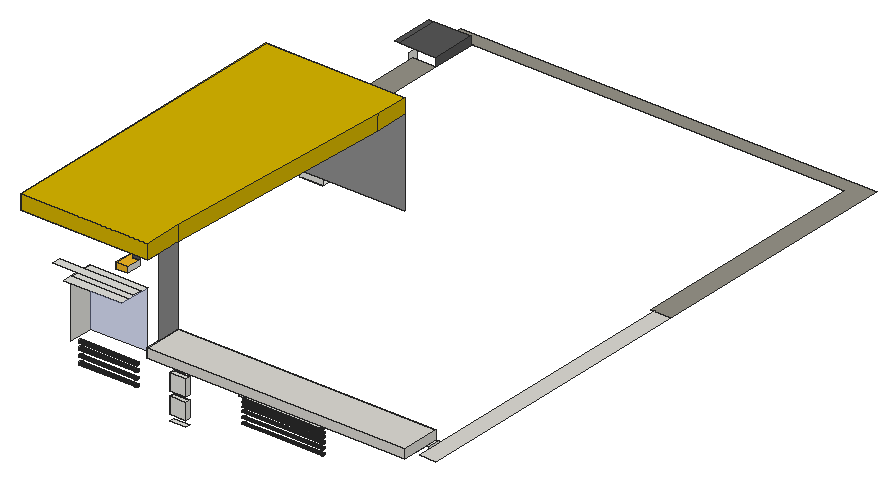
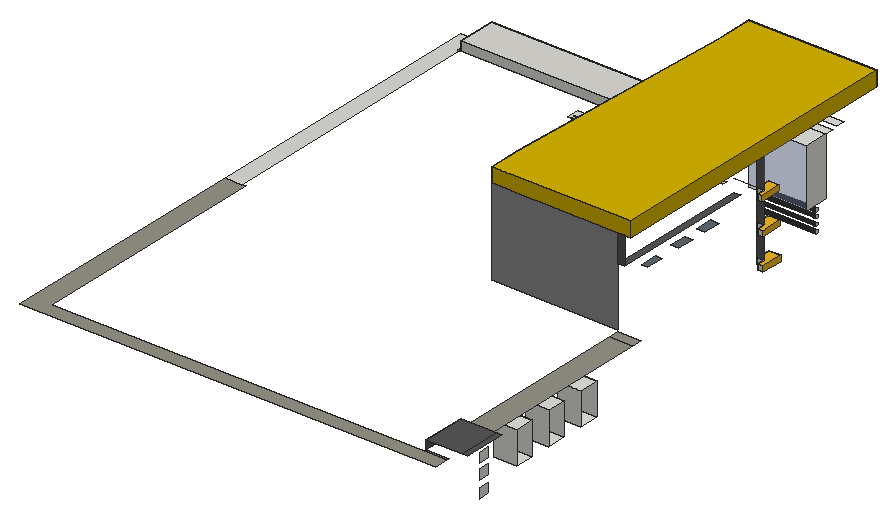
# SketchUp Ruby script. Lengths in inches.
U = 1.inch
M = Sketchup.active_model
def pt(a) = Geom::Point3d.new(a.map { |v| v * U })
def face(e, loops, mat)
  f = e.add_face(loops[0].map { |a| pt(a) })
  loops[1..].each { |l| e.add_face(l.map { |a| pt(a) }).erase! }
  f.material = f.back_material = mat if mat
  f
end
# faces: each face lists its corners as indices into pts; further lists are holes
def faces(e, pts, list, mat = nil) = list.each { |f| face(e, (f[0].is_a?(Array) ? f : [f]).map { |l| l.map { |i| pts[i] } }, mat) }
# xy, xz, yz: faces in a plane at the given z, y or x. An outline is a flat list of corners, or four numbers for a rectangle; further outlines are holes
def ring(l) = l.size == 4 ? [[l[0], l[1]], [l[2], l[1]], [l[2], l[3]], [l[0], l[3]]] : l.each_slice(2).to_a
def flat(e, list, mat, &to3) = list.each { |f| face(e, (f[0].is_a?(Array) ? f : [f]).map { |l| ring(l).map { |u, v| to3.(u, v) } }, mat) }
def xy(e, z, list, mat = nil) = flat(e, list, mat) { |x, y| [x, y, z] }
def xz(e, y, list, mat = nil) = flat(e, list, mat) { |x, z| [x, y, z] }
def yz(e, x, list, mat = nil) = flat(e, list, mat) { |y, z| [x, y, z] }
def lines(e, pts, list) = list.each { |a, b| e.add_line(pt(pts[a]), pt(pts[b])) }
# prism: a flat outline (further loops are holes) pulled along v
def prism(e, loops, v, mat = nil)
  f = face(e, loops, mat); d = Geom::Vector3d.new(v.map { |x| x * U })
  f.pushpull(f.normal.samedirection?(d) ? d.length : -d.length)
end
def box(e, o, s, mat = nil) = prism(e, [[o, [o[0] + s[0], o[1], o[2]], [o[0] + s[0], o[1] + s[1], o[2]], [o[0], o[1] + s[1], o[2]]]], [0, 0, s[2]], mat)
def at(x, y, z, deg = 0) = Geom::Transformation.translation(pt([x, y, z])) * Geom::Transformation.rotation(ORIGIN, Z_AXIS, deg.degrees)
def axes(o, x, y, z) = Geom::Transformation.new([*x, 0, *y, 0, *z, 0, *pt(o).to_a, 1])
def part(name) = M.definitions.add(name)
# library, detail: a bought-in or finely detailed component or shape, given as its bounding box
def library(name, o, s) = part(name).tap { |d| box(d.entities, o, s) }
def detail(e, o, s) = box(e.add_group.entities, o, s)
def put(e, d, t, mat = nil) = e.add_instance(d, t).tap { |i| i.material = mat if mat }
def group(e, t, mat = nil) = e.add_group.tap { |g| g.transformation = t; g.material = mat if mat }.entities
root = M.entities
M.materials.add("[0045_Goldenrod]").color = [239, 181, 35]
M.materials.add("[0046_Gold]1").color = [214, 180, 0]
M.materials.add("[Color M04]").color = [142, 142, 142]
M.materials.add("[Color M06]").color = [86, 86, 86]
M.materials.add("[Color M07]").color = [58, 58, 58]
M.materials.add("[Formica Graystone]").color = [149, 146, 135]
M.materials.add("[Formica Speckled Grey]").color = [94, 105, 111]
M.materials.add("[Terrazzo Tile Light]").color = [219, 217, 210]
M.materials.add("[Translucent Glass Sky Reflection]").color = [126, 138, 183]
M.materials["[Translucent Glass Sky Reflection]"].alpha = 0.52
box(root,[220.22,108.25,417.34],[19.63,5.9375,19.63])
box(root,[220.22,108.25,443.22],[19.63,5.9375,19.62])
xy(root,409.78,[[220.22,108.25,239.85,114.1875]])
xy(root,414.79,[[25.28,551.74,53.375,575.93],[25.28,600.93,53.375,625.12],[25.28,649.81,53.375,673.99]])
xy(root,445.19,[[[280.22,138.52,379.09,153.42],[329.08,144.78,329.38,144.82,329.67,144.9375,329.91,145.125,330.1,145.37,330.22,145.66,330.26,145.96,330.22,146.27,330.1,146.56,329.91,146.8,329.67,146.99,329.38,147.11,329.08,147.15,328.77,147.11,328.48,146.99,328.24,146.8,328.05,146.56,327.93,146.27,327.89,145.96,327.93,145.66,328.05,145.37,328.24,145.125,328.48,144.9375,328.77,144.82]]])
xy(root,449.66,[[38.625,253.03,38.625,280.03,45.3125,280.03,45.3125,270.46,53.375,270.46,53.375,253.03]],"[0045_Goldenrod]")
xy(root,454.59,[[25.28,551.74,53.375,575.93],[25.28,600.93,53.375,625.12],[25.28,649.81,53.375,673.99]])
xy(root,456.47,[[38.625,253.03,53.375,253.03,53.375,270.46,45.3125,270.46,45.3125,280.03,38.625,280.03]],"[0045_Goldenrod]")
xy(root,468.5,[[25.28,483.625,53.375,495.58],[509.21,483.625,533.375,483.625,533.375,797.6875,25.28,797.6875,25.28,779.875,509.21,779.875],[25.28,495.58,53.375,724.47],[25.28,777.2,53.375,779.875]],"[Formica Graystone]")
xy(root,468.5,[[513.45,123.625,533.375,483.625]],"[Terrazzo Tile Light]")
xy(root,471,[[194.63,105.9375,276.16,114.1875],[276.16,105.9375,276.16,138.52,385.17,138.52,385.17,125.375,418.48,125.375,418.48,138.52,435.42,138.52,435.42,125.375,467.86,125.375,467.86,138.52,510.34,138.52,510.34,105.9375],[194.63,114.1875,276.16,123.625],[194.63,123.625,276.16,153.42],[385.17,125.375,418.48,138.52],
  [435.42,125.375,467.86,138.52],[276.16,138.52,510.34,153.42],[510.34,138.52,513.45,153.42]])
xy(root,479.1875,[[2.5625,724.47,8.375,777.2],[8.375,724.47,53.375,777.2]],"[Color M06]")
xy(root,481.9375,[[194.63,105.9375,510.34,153.42]],"[Terrazzo Tile Light]")
xy(root,488.34,[[39.4375,253.03,39.4375,280.03,45.3125,280.03,45.3125,270.46,53.375,270.46,53.375,253.03]],"[0045_Goldenrod]")
xy(root,495.16,[[39.4375,253.03,53.375,253.03,53.375,270.46,45.3125,270.46,45.3125,280.03,39.4375,280.03]],"[0045_Goldenrod]")
xy(root,515.31,[[87.31,112.625,158.23,123.625],[87.31,123.625,158.23,152]])
xy(root,519.67,[[53.375,329.18,63.8125,350.43],[53.375,369.37,62.6875,390.62],[53.375,417,60.4375,438.25]],"[Formica Speckled Grey]")
xy(root,526.41,[[40.5,253.03,40.5,280.03,45.3125,280.03,45.3125,270.46,53.375,270.46,53.375,253.03]],"[0045_Goldenrod]")
xy(root,529.3125,[[73.3,112.625,172.24,123.625]])
xy(root,533.22,[[40.5,253.03,53.375,253.03,53.375,270.46,45.3125,270.46,45.3125,280.03,40.5,280.03]],"[0045_Goldenrod]")
xy(root,543.2,[[45.3125,306.125,53.375,483.625]],"[Color M06]")
xy(root,577.3125,[[38.125,107.4375,53.375,136.75],[53.375,107.4375,194.63,123.625],[53.375,123.625,53.375,483.625,73.3,483.625,73.3,463.7,208.03,463.7,208.03,442.17,194.63,153.42,194.63,123.625],[38.125,136.75,45.75,151.32],[45.75,136.75,53.375,151.32],
  [38.125,151.32,53.375,169.81],[38.125,169.81,45.75,184.38],[45.75,169.81,53.375,184.38],[38.125,184.38,53.375,206.12],[38.125,206.12,45.75,220.7],
  [45.75,206.12,53.375,220.7],[38.125,220.7,53.375,270.46],[38.125,270.46,45.3125,483.625],[45.3125,270.46,53.375,483.625],[73.3,463.7,208.03,483.625]])
xy(root,595.5,[[38.125,107.4375,194.63,107.4375,194.63,153.42,208.03,442.17,208.03,483.625,38.125,483.625]],"[0046_Gold]1")
xz(root,105.9375,[[194.63,471,510.34,481.9375]],"[Terrazzo Tile Light]")
xz(root,107.4375,[[38.125,577.3125,194.63,595.5]],"[0046_Gold]1")
xz(root,152,[[87.31,444.16,158.23,515.31]],"[Translucent Glass Sky Reflection]")
xz(root,153.42,[[194.63,471,510.34,481.9375]])
xz(root,253.03,[[38.625,449.66,53.375,456.47],[39.4375,488.34,53.375,495.16],[40.5,526.41,53.375,533.22]],"[0045_Goldenrod]")
xz(root,270.46,[[45.3125,449.66,53.375,456.47],[45.3125,488.34,53.375,495.16],[45.3125,526.41,53.375,533.22]])
xz(root,270.46,[[45.3125,456.47,53.375,488.34],[45.3125,495.16,53.375,526.41],[45.3125,533.22,53.375,577.3125]],"[Color M06]")
xz(root,280.03,[[38.625,449.66,45.3125,456.47],[39.4375,488.34,45.3125,495.16],[40.5,526.41,45.3125,533.22]])
xz(root,483.625,[[38.125,577.3125,208.03,595.5]],"[0046_Gold]1")
xz(root,483.625,[[53.375,471,208.03,577.3125]],"[Color M04]")
xz(root,483.625,[[45.3125,543.2,53.375,577.3125]],"[Color M06]")
xz(root,551.74,[[25.28,414.79,53.375,454.59]])
xz(root,575.93,[[25.28,414.79,53.375,454.59]])
xz(root,600.93,[[25.28,414.79,53.375,454.59]])
xz(root,625.12,[[25.28,414.79,53.375,454.59]])
xz(root,649.81,[[25.28,414.79,53.375,454.59]])
xz(root,673.99,[[25.28,414.79,53.375,454.59]])
yz(root,2.5625,[[745.75,424.57,759.0625,436.32],[745.75,444.94,759.0625,456.69],[745.75,463.32,759.0625,475.07]])
yz(root,38.125,[[107.4375,577.3125,483.625,595.5]],"[0046_Gold]1")
yz(root,38.625,[[253.03,449.66,280.03,456.47]],"[0045_Goldenrod]")
yz(root,39.4375,[[253.03,488.34,280.03,495.16]],"[0045_Goldenrod]")
yz(root,40.5,[[253.03,526.41,280.03,533.22]],"[0045_Goldenrod]")
yz(root,45.3125,[[270.46,449.66,280.03,456.47],[270.46,488.34,280.03,495.16],[270.46,526.41,280.03,533.22]])
yz(root,53.375,[[253.03,449.66,270.46,456.47],[253.03,488.34,270.46,495.16],[253.03,526.41,270.46,533.22]])
yz(root,53.375,[[724.47,468.5,777.2,479.1875]],"[Color M06]")
yz(root,87.31,[[136.99,412.55,136.55,412.61,136.14,412.78,135.79,413.05,135.52,413.4,135.36,413.81,135.3,414.24,135.36,414.68,135.52,415.09,135.79,415.44,136.14,415.7,136.55,415.87,136.99,415.93,137.42,415.87,137.83,415.7,138.18,415.44,138.45,415.09,138.62,414.68,138.67,414.24,138.62,413.81,138.45,413.4,138.18,413.05,137.83,412.78,137.42,412.61],[136.99,420.74,136.55,420.8,136.14,420.97,135.79,421.24,135.52,421.59,135.36,421.99,135.3,422.43,135.36,422.87,135.52,423.27,135.79,423.62,136.14,423.89,136.55,424.06,136.99,424.12,137.42,424.06,137.83,423.89,138.18,423.62,138.45,423.27,138.62,422.87,138.67,422.43,138.62,421.99,138.45,421.59,138.18,421.24,137.83,420.97,137.42,420.8],[136.99,429.05,136.55,429.11,136.14,429.28,135.79,429.55,135.52,429.9,135.36,430.31,135.3,430.74,135.36,431.18,135.52,431.59,135.79,431.94,136.14,432.2,136.55,432.37,136.99,432.43,137.42,432.37,137.83,432.2,138.18,431.94,138.45,431.59,138.62,431.18,138.67,430.74,138.62,430.31,138.45,429.9,138.18,429.55,137.83,429.28,137.42,429.11],[136.99,436.55,136.55,436.61,136.14,436.78,135.79,437.05,135.52,437.4,135.36,437.81,135.3,438.24,135.36,438.68,135.52,439.09,135.79,439.44,136.14,439.7,136.55,439.87,136.99,439.93,137.42,439.87,137.83,439.7,138.18,439.44,138.45,439.09,138.62,438.68,138.67,438.24,138.62,437.81,138.45,437.4,138.18,437.05,137.83,436.78,137.42,436.61],[123.625,444.16,152,515.31]])
yz(root,194.63,[[123.625,471,153.42,481.9375]])
yz(root,194.63,[[107.4375,577.3125,153.42,595.5]],"[0046_Gold]1")
yz(root,194.63,[[123.625,481.9375,153.42,577.3125]],"[Color M04]")
yz(root,194.63,[[105.9375,471,123.625,481.9375]],"[Terrazzo Tile Light]")
yz(root,208.03,[[442.17,577.3125,483.625,595.5]],"[0046_Gold]1")
yz(root,280.22,[[145.61,411.18,145.26,411.23,144.93,411.37,144.64,411.59,144.42,411.87,144.29,412.2,144.24,412.56,144.29,412.92,144.42,413.25,144.64,413.53,144.93,413.75,145.26,413.89,145.61,413.93,145.97,413.89,146.3,413.75,146.59,413.53,146.81,413.25,146.94,412.92,146.99,412.56,146.94,412.2,146.81,411.87,146.59,411.59,146.3,411.37,145.97,411.23],[145.61,417.75,145.26,417.79,144.93,417.93,144.64,418.15,144.42,418.43,144.29,418.77,144.24,419.12,144.29,419.48,144.42,419.81,144.64,420.09,144.93,420.3125,145.26,420.45,145.61,420.5,145.97,420.45,146.3,420.3125,146.59,420.09,146.81,419.81,146.94,419.48,146.99,419.12,146.94,418.77,146.81,418.43,146.59,418.15,146.3,417.93,145.97,417.79],[145.61,424.12,145.26,424.17,144.93,424.31,144.64,424.52,144.42,424.81,144.29,425.14,144.24,425.5,144.29,425.85,144.42,426.18,144.64,426.47,144.93,426.6875,145.26,426.83,145.61,426.87,145.97,426.83,146.3,426.6875,146.59,426.47,146.81,426.18,146.94,425.85,146.99,425.5,146.94,425.14,146.81,424.81,146.59,424.52,146.3,424.31,145.97,424.17],[145.73,429.69,145.38,429.74,145.05,429.875,144.76,430.09,144.54,430.38,144.41,430.71,144.36,431.07,144.41,431.42,144.54,431.75,144.76,432.04,145.05,432.26,145.38,432.39,145.73,432.44,146.09,432.39,146.42,432.26,146.71,432.04,146.92,431.75,147.0625,431.42,147.11,431.07,147.0625,430.71,146.92,430.38,146.71,430.09,146.42,429.875,146.09,429.74],[145.73,434.63,145.38,434.67,145.05,434.8125,144.76,435.03,144.54,435.32,144.41,435.65,144.36,436,144.41,436.36,144.54,436.69,144.76,436.97,145.05,437.19,145.38,437.33,145.73,437.38,146.09,437.33,146.42,437.19,146.71,436.97,146.92,436.69,147.0625,436.36,147.11,436,147.0625,435.65,146.92,435.32,146.71,435.03,146.42,434.8125,146.09,434.67],
  [145.73,439.94,145.38,439.99,145.05,440.125,144.76,440.34,144.54,440.63,144.41,440.96,144.36,441.32,144.41,441.67,144.54,442,144.76,442.29,145.05,442.51,145.38,442.64,145.73,442.69,146.09,442.64,146.42,442.51,146.71,442.29,146.92,442,147.0625,441.67,147.11,441.32,147.0625,440.96,146.92,440.63,146.71,440.34,146.42,440.125,146.09,439.99]])
yz(root,510.34,[[105.9375,471,153.42,481.9375]],"[Terrazzo Tile Light]")
yz(root,513.45,[[138.52,468.5,153.42,471]])
p = [[280.22,144.93,411.37],[280.22,145.26,411.23],[379.09,145.26,411.23],[379.09,144.93,411.37],[280.22,145.61,411.18],[379.09,145.61,411.18],
  [280.22,145.97,411.23],[379.09,145.97,411.23],[280.22,146.3,411.37],[379.09,146.3,411.37],[280.22,144.64,411.59],[379.09,144.64,411.59],
  [280.22,146.59,411.59],[379.09,146.59,411.59],[280.22,144.42,411.87],[379.09,144.42,411.87],[280.22,146.81,411.87],[379.09,146.81,411.87],
  [280.22,144.29,412.2],[379.09,144.29,412.2],[280.22,146.94,412.2],[379.09,146.94,412.2],[280.22,144.24,412.56],[379.09,144.24,412.56],
  [280.22,146.99,412.56],[379.09,146.99,412.56],[87.31,136.14,412.78],[87.31,136.55,412.61],[158.23,136.55,412.61],[158.23,136.14,412.78],
  [87.31,136.99,412.55],[158.23,136.99,412.55],[87.31,137.42,412.61],[158.23,137.42,412.61],[87.31,137.83,412.78],[158.23,137.83,412.78],
  [280.22,144.29,412.92],[379.09,144.29,412.92],[280.22,146.94,412.92],[379.09,146.94,412.92],[87.31,135.79,413.05],[158.23,135.79,413.05],
  [87.31,138.18,413.05],[158.23,138.18,413.05],[280.22,144.42,413.25],[379.09,144.42,413.25],[280.22,146.81,413.25],[379.09,146.81,413.25],
  [87.31,135.52,413.4],[158.23,135.52,413.4],[87.31,138.45,413.4],[158.23,138.45,413.4],[280.22,144.64,413.53],[379.09,144.64,413.53],
  [280.22,146.59,413.53],[379.09,146.59,413.53],[87.31,135.36,413.81],[158.23,135.36,413.81],[87.31,138.62,413.81],[158.23,138.62,413.81],
  [280.22,144.93,413.75],[379.09,144.93,413.75],[280.22,146.3,413.75],[379.09,146.3,413.75],[87.31,135.3,414.24],[158.23,135.3,414.24],
  [87.31,138.67,414.24],[158.23,138.67,414.24],[280.22,145.26,413.89],[379.09,145.26,413.89],[280.22,145.97,413.89],[379.09,145.97,413.89],
  [280.22,145.61,413.93],[379.09,145.61,413.93],[87.31,135.36,414.68],[158.23,135.36,414.68],[87.31,138.62,414.68],[158.23,138.62,414.68],
  [87.31,135.52,415.09],[158.23,135.52,415.09],[87.31,138.45,415.09],[158.23,138.45,415.09],[87.31,135.79,415.44],[158.23,135.79,415.44],
  [87.31,138.18,415.44],[158.23,138.18,415.44],[87.31,136.14,415.7],[158.23,136.14,415.7],[87.31,137.83,415.7],[158.23,137.83,415.7],
  [87.31,136.55,415.87],[158.23,136.55,415.87],[87.31,137.42,415.87],[158.23,137.42,415.87],[87.31,136.99,415.93],[158.23,136.99,415.93],
  [280.22,145.26,417.79],[280.22,145.61,417.75],[379.09,145.61,417.75],[379.09,145.26,417.79],[280.22,145.97,417.79],[379.09,145.97,417.79],
  [280.22,144.93,417.93],[379.09,144.93,417.93],[280.22,146.3,417.93],[379.09,146.3,417.93],[280.22,144.64,418.15],[379.09,144.64,418.15],
  [280.22,146.59,418.15],[379.09,146.59,418.15],[280.22,144.42,418.43],[379.09,144.42,418.43],[280.22,146.81,418.43],[379.09,146.81,418.43],
  [280.22,144.29,418.77],[379.09,144.29,418.77],[280.22,146.94,418.77],[379.09,146.94,418.77],[280.22,144.24,419.12],[379.09,144.24,419.12],
  [280.22,146.99,419.12],[379.09,146.99,419.12],[280.22,144.29,419.48],[379.09,144.29,419.48],[280.22,146.94,419.48],[379.09,146.94,419.48],
  [280.22,144.42,419.81],[379.09,144.42,419.81],[280.22,146.81,419.81],[379.09,146.81,419.81],[280.22,144.64,420.09],[379.09,144.64,420.09],
  [280.22,146.59,420.09],[379.09,146.59,420.09],[280.22,144.93,420.3125],[379.09,144.93,420.3125],[280.22,146.3,420.3125],[379.09,146.3,420.3125],
  [280.22,145.26,420.45],[379.09,145.26,420.45],[280.22,145.97,420.45],[379.09,145.97,420.45],[280.22,145.61,420.5],[379.09,145.61,420.5],
  [87.31,136.55,420.8],[87.31,136.99,420.74],[158.23,136.99,420.74],[158.23,136.55,420.8],[87.31,137.42,420.8],[158.23,137.42,420.8],
  [87.31,136.14,420.97],[158.23,136.14,420.97],[87.31,137.83,420.97],[158.23,137.83,420.97],[87.31,135.79,421.24],[158.23,135.79,421.24],
  [87.31,138.18,421.24],[158.23,138.18,421.24],[87.31,135.52,421.59],[158.23,135.52,421.59],[87.31,138.45,421.59],[158.23,138.45,421.59],
  [87.31,135.36,421.99],[158.23,135.36,421.99],[87.31,138.62,421.99],[158.23,138.62,421.99],[87.31,135.3,422.43],[158.23,135.3,422.43],
  [87.31,138.67,422.43],[158.23,138.67,422.43],[87.31,135.36,422.87],[158.23,135.36,422.87],[87.31,138.62,422.87],[158.23,138.62,422.87],
  [87.31,135.52,423.27],[158.23,135.52,423.27],[87.31,138.45,423.27],[158.23,138.45,423.27],[87.31,135.79,423.62],[158.23,135.79,423.62],
  [87.31,138.18,423.62],[158.23,138.18,423.62],[87.31,136.14,423.89],[158.23,136.14,423.89],[87.31,137.83,423.89],[158.23,137.83,423.89],
  [87.31,136.55,424.06],[158.23,136.55,424.06],[87.31,137.42,424.06],[158.23,137.42,424.06],[87.31,136.99,424.12],[158.23,136.99,424.12],
  [280.22,145.26,424.17],[280.22,145.61,424.12],[379.09,145.61,424.12],[379.09,145.26,424.17],[280.22,145.97,424.17],[379.09,145.97,424.17],
  [280.22,144.93,424.31],[379.09,144.93,424.31],[280.22,146.3,424.31],[379.09,146.3,424.31],[280.22,144.64,424.52],[379.09,144.64,424.52],
  [280.22,146.59,424.52],[379.09,146.59,424.52],[280.22,144.42,424.81],[379.09,144.42,424.81],[280.22,146.81,424.81],[379.09,146.81,424.81],
  [280.22,144.29,425.14],[379.09,144.29,425.14],[280.22,146.94,425.14],[379.09,146.94,425.14],[280.22,144.24,425.5],[379.09,144.24,425.5],
  [280.22,146.99,425.5],[379.09,146.99,425.5],[280.22,144.29,425.85],[379.09,144.29,425.85],[280.22,146.94,425.85],[379.09,146.94,425.85],
  [280.22,144.42,426.18],[379.09,144.42,426.18],[280.22,146.81,426.18],[379.09,146.81,426.18],[280.22,144.64,426.47],[379.09,144.64,426.47],
  [280.22,146.59,426.47],[379.09,146.59,426.47],[280.22,144.93,426.6875],[379.09,144.93,426.6875],[280.22,146.3,426.6875],[379.09,146.3,426.6875],
  [280.22,145.26,426.83],[379.09,145.26,426.83],[280.22,145.97,426.83],[379.09,145.97,426.83],[280.22,145.61,426.87],[379.09,145.61,426.87],
  [87.31,136.14,429.28],[87.31,136.55,429.11],[158.23,136.55,429.11],[158.23,136.14,429.28],[87.31,136.99,429.05],[158.23,136.99,429.05],
  [87.31,137.42,429.11],[158.23,137.42,429.11],[87.31,137.83,429.28],[158.23,137.83,429.28],[87.31,135.79,429.55],[158.23,135.79,429.55],
  [87.31,138.18,429.55],[158.23,138.18,429.55],[87.31,135.52,429.9],[158.23,135.52,429.9],[87.31,138.45,429.9],[158.23,138.45,429.9],
  [280.22,145.05,429.875],[280.22,145.38,429.74],[379.09,145.38,429.74],[379.09,145.05,429.875],[280.22,145.73,429.69],[379.09,145.73,429.69],
  [280.22,146.09,429.74],[379.09,146.09,429.74],[280.22,146.42,429.875],[379.09,146.42,429.875],[87.31,135.36,430.31],[158.23,135.36,430.31],
  [87.31,138.62,430.31],[158.23,138.62,430.31],[280.22,144.76,430.09],[379.09,144.76,430.09],[280.22,146.71,430.09],[379.09,146.71,430.09],
  [280.22,144.54,430.38],[379.09,144.54,430.38],[280.22,146.92,430.38],[379.09,146.92,430.38],[87.31,135.3,430.74],[158.23,135.3,430.74],
  [87.31,138.67,430.74],[158.23,138.67,430.74],[280.22,144.41,430.71],[379.09,144.41,430.71],[280.22,147.0625,430.71],[379.09,147.0625,430.71],
  [87.31,135.36,431.18],[158.23,135.36,431.18],[87.31,138.62,431.18],[158.23,138.62,431.18],[280.22,144.36,431.07],[379.09,144.36,431.07],
  [280.22,147.11,431.07],[379.09,147.11,431.07],[280.22,144.41,431.42],[379.09,144.41,431.42],[280.22,147.0625,431.42],[379.09,147.0625,431.42],
  [87.31,135.52,431.59],[158.23,135.52,431.59],[87.31,138.45,431.59],[158.23,138.45,431.59],[280.22,144.54,431.75],[379.09,144.54,431.75],
  [280.22,146.92,431.75],[379.09,146.92,431.75],[87.31,135.79,431.94],[158.23,135.79,431.94],[87.31,138.18,431.94],[158.23,138.18,431.94],
  [280.22,144.76,432.04],[379.09,144.76,432.04],[280.22,146.71,432.04],[379.09,146.71,432.04],[87.31,136.14,432.2],[158.23,136.14,432.2],
  [87.31,137.83,432.2],[158.23,137.83,432.2],[280.22,145.05,432.26],[379.09,145.05,432.26],[280.22,146.42,432.26],[379.09,146.42,432.26],
  [87.31,136.55,432.37],[158.23,136.55,432.37],[87.31,137.42,432.37],[158.23,137.42,432.37],[280.22,145.38,432.39],[379.09,145.38,432.39],
  [280.22,146.09,432.39],[379.09,146.09,432.39],[87.31,136.99,432.43],[158.23,136.99,432.43],[280.22,145.73,432.44],[379.09,145.73,432.44],
  [280.22,145.38,434.67],[280.22,145.73,434.63],[379.09,145.73,434.63],[379.09,145.38,434.67],[280.22,146.09,434.67],[379.09,146.09,434.67],
  [280.22,145.05,434.8125],[379.09,145.05,434.8125],[280.22,146.42,434.8125],[379.09,146.42,434.8125],[280.22,144.76,435.03],[379.09,144.76,435.03],
  [280.22,146.71,435.03],[379.09,146.71,435.03],[280.22,144.54,435.32],[379.09,144.54,435.32],[280.22,146.92,435.32],[379.09,146.92,435.32],
  [280.22,144.41,435.65],[379.09,144.41,435.65],[280.22,147.0625,435.65],[379.09,147.0625,435.65],[280.22,144.36,436],[379.09,144.36,436],
  [280.22,147.11,436],[379.09,147.11,436],[280.22,144.41,436.36],[379.09,144.41,436.36],[280.22,147.0625,436.36],[379.09,147.0625,436.36],
  [280.22,144.54,436.69],[379.09,144.54,436.69],[280.22,146.92,436.69],[379.09,146.92,436.69],[87.31,136.14,436.78],[87.31,136.55,436.61],
  [158.23,136.55,436.61],[158.23,136.14,436.78],[87.31,136.99,436.55],[158.23,136.99,436.55],[87.31,137.42,436.61],[158.23,137.42,436.61],
  [87.31,137.83,436.78],[158.23,137.83,436.78],[280.22,144.76,436.97],[379.09,144.76,436.97],[280.22,146.71,436.97],[379.09,146.71,436.97],
  [87.31,135.79,437.05],[158.23,135.79,437.05],[87.31,138.18,437.05],[158.23,138.18,437.05],[87.31,135.52,437.4],[158.23,135.52,437.4],
  [87.31,138.45,437.4],[158.23,138.45,437.4],[280.22,145.05,437.19],[379.09,145.05,437.19],[280.22,146.42,437.19],[379.09,146.42,437.19],
  [280.22,145.38,437.33],[379.09,145.38,437.33],[280.22,146.09,437.33],[379.09,146.09,437.33],[280.22,145.73,437.38],[379.09,145.73,437.38],
  [87.31,135.36,437.81],[158.23,135.36,437.81],[87.31,138.62,437.81],[158.23,138.62,437.81],[87.31,135.3,438.24],[158.23,135.3,438.24],
  [87.31,138.67,438.24],[158.23,138.67,438.24],[87.31,135.36,438.68],[158.23,135.36,438.68],[87.31,138.62,438.68],[158.23,138.62,438.68],
  [87.31,135.52,439.09],[158.23,135.52,439.09],[87.31,138.45,439.09],[158.23,138.45,439.09],[87.31,135.79,439.44],[158.23,135.79,439.44],
  [87.31,138.18,439.44],[158.23,138.18,439.44],[87.31,136.14,439.7],[158.23,136.14,439.7],[87.31,137.83,439.7],[158.23,137.83,439.7],
  [87.31,136.55,439.87],[158.23,136.55,439.87],[87.31,137.42,439.87],[158.23,137.42,439.87],[87.31,136.99,439.93],[158.23,136.99,439.93],
  [280.22,145.38,439.99],[280.22,145.73,439.94],[379.09,145.73,439.94],[379.09,145.38,439.99],[280.22,146.09,439.99],[379.09,146.09,439.99],
  [280.22,145.05,440.125],[379.09,145.05,440.125],[280.22,146.42,440.125],[379.09,146.42,440.125],[280.22,144.76,440.34],[379.09,144.76,440.34],
  [280.22,146.71,440.34],[379.09,146.71,440.34],[280.22,144.54,440.63],[379.09,144.54,440.63],[280.22,146.92,440.63],[379.09,146.92,440.63],
  [280.22,144.41,440.96],[379.09,144.41,440.96],[280.22,147.0625,440.96],[379.09,147.0625,440.96],[280.22,144.36,441.32],[379.09,144.36,441.32],
  [280.22,147.11,441.32],[379.09,147.11,441.32],[280.22,144.41,441.67],[379.09,144.41,441.67],[280.22,147.0625,441.67],[379.09,147.0625,441.67],
  [280.22,144.54,442],[379.09,144.54,442],[280.22,146.92,442],[379.09,146.92,442],[280.22,144.76,442.29],[379.09,144.76,442.29],
  [280.22,146.71,442.29],[379.09,146.71,442.29],[280.22,145.05,442.51],[379.09,145.05,442.51],[280.22,146.42,442.51],[379.09,146.42,442.51],
  [280.22,145.38,442.64],[379.09,145.38,442.64],[280.22,146.09,442.64],[379.09,146.09,442.64],[280.22,145.73,442.69],[379.09,145.73,442.69],
  [194.63,153.42,577.3125],[208.03,442.17,577.3125],[208.03,442.17,595.5],[194.63,153.42,595.5],[53.375,270.46,533.22],[82.3125,270.46,533.22]]
faces(root,p,[[0,1,2,3],[1,4,5,2],[4,6,7,5],[6,8,9,7],[10,0,3,11],[8,12,13,9],[14,10,11,15],[12,16,17,13],
  [18,14,15,19],[16,20,21,17],[22,18,19,23],[20,24,25,21],[26,27,28,29],[27,30,31,28],[30,32,33,31],[32,34,35,33],
  [36,22,23,37],[24,38,39,25],[40,26,29,41],[34,42,43,35],[44,36,37,45],[38,46,47,39],[48,40,41,49],[42,50,51,43],
  [52,44,45,53],[46,54,55,47],[56,48,49,57],[50,58,59,51],[60,52,53,61],[54,62,63,55],[64,56,57,65],[58,66,67,59],
  [68,60,61,69],[62,70,71,63],[72,68,69,73],[70,72,73,71],[74,64,65,75],[66,76,77,67],[78,74,75,79],[76,80,81,77],
  [82,78,79,83],[80,84,85,81],[86,82,83,87],[84,88,89,85],[90,86,87,91],[88,92,93,89],[94,90,91,95],[92,94,95,93],
  [96,97,98,99],[97,100,101,98],[102,96,99,103],[100,104,105,101],[106,102,103,107],[104,108,109,105],[110,106,107,111],[108,112,113,109],
  [114,110,111,115],[112,116,117,113],[118,114,115,119],[116,120,121,117],[122,118,119,123],[120,124,125,121],[126,122,123,127],[124,128,129,125],
  [130,126,127,131],[128,132,133,129],[134,130,131,135],[132,136,137,133],[138,134,135,139],[136,140,141,137],[142,138,139,143],[140,142,143,141],
  [144,145,146,147],[145,148,149,146],[150,144,147,151],[148,152,153,149],[154,150,151,155],[152,156,157,153],[158,154,155,159],[156,160,161,157],
  [162,158,159,163],[160,164,165,161],[166,162,163,167],[164,168,169,165],[170,166,167,171],[168,172,173,169],[174,170,171,175],[172,176,177,173],
  [178,174,175,179],[176,180,181,177],[182,178,179,183],[180,184,185,181],[186,182,183,187],[184,188,189,185],[190,186,187,191],[188,190,191,189],
  [192,193,194,195],[193,196,197,194],[198,192,195,199],[196,200,201,197],[202,198,199,203],[200,204,205,201],[206,202,203,207],[204,208,209,205],
  [210,206,207,211],[208,212,213,209],[214,210,211,215],[212,216,217,213],[218,214,215,219],[216,220,221,217],[222,218,219,223],[220,224,225,221],
  [226,222,223,227],[224,228,229,225],[230,226,227,231],[228,232,233,229],[234,230,231,235],[232,236,237,233],[238,234,235,239],[236,238,239,237],
  [240,241,242,243],[241,244,245,242],[244,246,247,245],[246,248,249,247],[250,240,243,251],[248,252,253,249],[254,250,251,255],[252,256,257,253],
  [258,259,260,261],[259,262,263,260],[262,264,265,263],[264,266,267,265],[268,254,255,269],[256,270,271,257],[272,258,261,273],[266,274,275,267],
  [276,272,273,277],[274,278,279,275],[280,268,269,281],[270,282,283,271],[284,276,277,285],[278,286,287,279],[288,280,281,289],[282,290,291,283],
  [292,284,285,293],[286,294,295,287],[296,292,293,297],[294,298,299,295],[300,288,289,301],[290,302,303,291],[304,296,297,305],[298,306,307,299],
  [308,300,301,309],[302,310,311,303],[312,304,305,313],[306,314,315,307],[316,308,309,317],[310,318,319,311],[320,312,313,321],[314,322,323,315],
  [324,316,317,325],[318,326,327,319],[328,320,321,329],[322,330,331,323],[332,324,325,333],[326,332,333,327],[334,328,329,335],[330,334,335,331],
  [336,337,338,339],[337,340,341,338],[342,336,339,343],[340,344,345,341],[346,342,343,347],[344,348,349,345],[350,346,347,351],[348,352,353,349],
  [354,350,351,355],[352,356,357,353],[358,354,355,359],[356,360,361,357],[362,358,359,363],[360,364,365,361],[366,362,363,367],[364,368,369,365],
  [370,371,372,373],[371,374,375,372],[374,376,377,375],[376,378,379,377],[380,366,367,381],[368,382,383,369],[384,370,373,385],[378,386,387,379],
  [388,384,385,389],[386,390,391,387],[392,380,381,393],[382,394,395,383],[396,392,393,397],[394,398,399,395],[400,396,397,401],[398,400,401,399],
  [402,388,389,403],[390,404,405,391],[406,402,403,407],[404,408,409,405],[410,406,407,411],[408,412,413,409],[414,410,411,415],[412,416,417,413],
  [418,414,415,419],[416,420,421,417],[422,418,419,423],[420,424,425,421],[426,422,423,427],[424,428,429,425],[430,426,427,431],[428,430,431,429],
  [432,433,434,435],[433,436,437,434],[438,432,435,439],[436,440,441,437],[442,438,439,443],[440,444,445,441],[446,442,443,447],[444,448,449,445],
  [450,446,447,451],[448,452,453,449],[454,450,451,455],[452,456,457,453],[458,454,455,459],[456,460,461,457],[462,458,459,463],[460,464,465,461],
  [466,462,463,467],[464,468,469,465],[470,466,467,471],[468,472,473,469],[474,470,471,475],[472,476,477,473],[478,474,475,479],[476,478,479,477]],"[Color M07]")
faces(root,p,[[480,481,482,483]],"[0046_Gold]1")
lines(root,p,[[484,485]])
